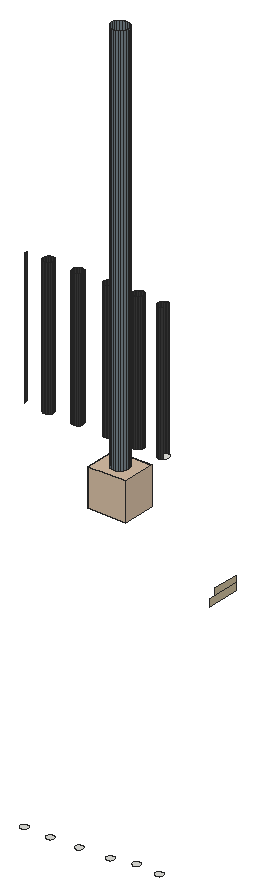
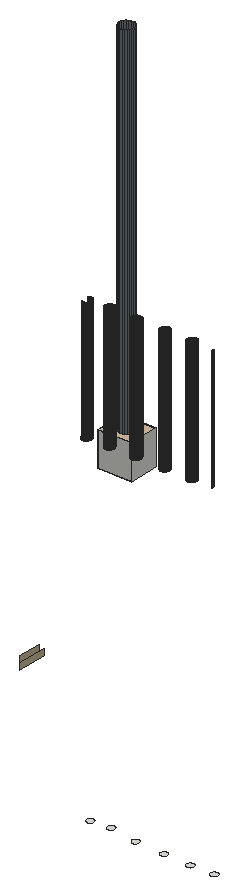
# SketchUp Ruby script. Lengths in inches.
U = 1.inch
M = Sketchup.active_model
def pt(a) = Geom::Point3d.new(a.map { |v| v * U })
def face(e, loops, mat)
  f = e.add_face(loops[0].map { |a| pt(a) })
  loops[1..].each { |l| e.add_face(l.map { |a| pt(a) }).erase! }
  f.material = f.back_material = mat if mat
  f
end
# faces: each face lists its corners as indices into pts; further lists are holes
def faces(e, pts, list, mat = nil) = list.each { |f| face(e, (f[0].is_a?(Array) ? f : [f]).map { |l| l.map { |i| pts[i] } }, mat) }
# xy, xz, yz: faces in a plane at the given z, y or x. An outline is a flat list of corners, or four numbers for a rectangle; further outlines are holes
def ring(l) = l.size == 4 ? [[l[0], l[1]], [l[2], l[1]], [l[2], l[3]], [l[0], l[3]]] : l.each_slice(2).to_a
def flat(e, list, mat, &to3) = list.each { |f| face(e, (f[0].is_a?(Array) ? f : [f]).map { |l| ring(l).map { |u, v| to3.(u, v) } }, mat) }
def xy(e, z, list, mat = nil) = flat(e, list, mat) { |x, y| [x, y, z] }
def xz(e, y, list, mat = nil) = flat(e, list, mat) { |x, z| [x, y, z] }
def yz(e, x, list, mat = nil) = flat(e, list, mat) { |y, z| [x, y, z] }
def lines(e, pts, list) = list.each { |a, b| e.add_line(pt(pts[a]), pt(pts[b])) }
# prism: a flat outline (further loops are holes) pulled along v
def prism(e, loops, v, mat = nil)
  f = face(e, loops, mat); d = Geom::Vector3d.new(v.map { |x| x * U })
  f.pushpull(f.normal.samedirection?(d) ? d.length : -d.length)
end
def box(e, o, s, mat = nil) = prism(e, [[o, [o[0] + s[0], o[1], o[2]], [o[0] + s[0], o[1] + s[1], o[2]], [o[0], o[1] + s[1], o[2]]]], [0, 0, s[2]], mat)
def at(x, y, z, deg = 0) = Geom::Transformation.translation(pt([x, y, z])) * Geom::Transformation.rotation(ORIGIN, Z_AXIS, deg.degrees)
def axes(o, x, y, z) = Geom::Transformation.new([*x, 0, *y, 0, *z, 0, *pt(o).to_a, 1])
def part(name) = M.definitions.add(name)
# library, detail: a bought-in or finely detailed component or shape, given as its bounding box
def library(name, o, s) = part(name).tap { |d| box(d.entities, o, s) }
def detail(e, o, s) = box(e.add_group.entities, o, s)
def put(e, d, t, mat = nil) = e.add_instance(d, t).tap { |i| i.material = mat if mat }
def group(e, t, mat = nil) = e.add_group.tap { |g| g.transformation = t; g.material = mat if mat }.entities
root = M.entities
M.materials.add("[Color M07]").color = [58, 58, 58]
M.materials.add("[Formica Laminate Light]").color = [213, 189, 164]
M.materials.add("[Formica Speckled Grey]").color = [112, 125, 132]
M.materials.add("[Quartz Light Brown]").color = [199, 184, 152]
xy(root,298.96,[[100.78,91.87,100.96,91.89,101.125,91.96,101.27,92.07,101.375,92.21,101.44,92.38,101.47,92.56,101.44,92.73,101.375,92.9,101.27,93.04,101.125,93.15,100.96,93.22,100.78,93.24,100.6,93.22,100.4375,93.15,100.29,93.04,100.18,92.9,100.12,92.73,100.09,92.56,100.12,92.38,100.18,92.21,100.29,92.07,100.4375,91.96,100.6,91.89]])
xy(root,299.02,[[95.78,91.87,95.96,91.89,96.125,91.96,96.27,92.07,96.375,92.21,96.44,92.38,96.47,92.56,96.44,92.73,96.375,92.9,96.27,93.04,96.125,93.15,95.96,93.22,95.78,93.24,95.6,93.22,95.4375,93.15,95.29,93.04,95.18,92.9,95.12,92.73,95.09,92.56,95.12,92.38,95.18,92.21,95.29,92.07,95.4375,91.96,95.6,91.89]])
xy(root,299.14,[[106.34,91.87,106.52,91.89,106.6875,91.96,106.83,92.07,106.9375,92.21,107.01,92.38,107.03,92.56,107.01,92.73,106.9375,92.9,106.83,93.04,106.6875,93.15,106.52,93.22,106.34,93.24,106.16,93.22,106,93.15,105.86,93.04,105.75,92.9,105.68,92.73,105.65,92.56,105.68,92.38,105.75,92.21,105.86,92.07,106,91.96,106.16,91.89]])
xy(root,299.39,[[112.34,91.87,112.52,91.89,112.6875,91.96,112.83,92.07,112.9375,92.21,113.01,92.38,113.03,92.56,113.01,92.73,112.9375,92.9,112.83,93.04,112.6875,93.15,112.52,93.22,112.34,93.24,112.16,93.22,112,93.15,111.86,93.04,111.75,92.9,111.68,92.73,111.65,92.56,111.68,92.38,111.75,92.21,111.86,92.07,112,91.96,112.16,91.89]])
xy(root,299.96,[[121.84,91.87,122.02,91.89,122.1875,91.96,122.33,92.07,122.4375,92.21,122.51,92.38,122.53,92.56,122.51,92.73,122.4375,92.9,122.33,93.04,122.1875,93.15,122.02,93.22,121.84,93.24,121.66,93.22,121.5,93.15,121.36,93.04,121.25,92.9,121.18,92.73,121.15,92.56,121.18,92.38,121.25,92.21,121.36,92.07,121.5,91.96,121.66,91.89]])
xy(root,300.16,[[117.47,91.87,117.64,91.89,117.8125,91.96,117.95,92.07,118.0625,92.21,118.13,92.38,118.15,92.56,118.13,92.73,118.0625,92.9,117.95,93.04,117.8125,93.15,117.64,93.22,117.47,93.24,117.29,93.22,117.125,93.15,116.98,93.04,116.87,92.9,116.8,92.73,116.78,92.56,116.8,92.38,116.87,92.21,116.98,92.07,117.125,91.96,117.29,91.89]])
xy(root,365.02,[[115.36,83.42,122.61,89.73]],"[Formica Laminate Light]")
xy(root,372.27,[[119,85,118.58,85.06,118.1875,85.22,117.85,85.48,117.59,85.82,117.43,86.21,117.375,86.63,117.43,87.05,117.59,87.44,117.85,87.78,118.1875,88.04,118.58,88.2,119,88.25,119.42,88.2,119.8125,88.04,120.15,87.78,120.41,87.44,120.57,87.05,120.625,86.63,120.57,86.21,120.41,85.82,120.15,85.48,119.8125,85.22,119.42,85.06],[100.02,92.0625,99.77,92.1,99.52,92.2,99.32,92.35,99.16,92.5625,99.06,92.8,99.02,93.0625,99.06,93.32,99.16,93.5625,99.32,93.77,99.52,93.93,99.77,94.03,100.02,94.0625,100.28,94.03,100.52,93.93,100.73,93.77,100.89,93.5625,100.99,93.32,101.02,93.0625,100.99,92.8,100.89,92.5625,100.73,92.35,100.52,92.2,100.28,92.1],[105.71,92.0625,105.45,92.1,105.21,92.2,105,92.35,104.85,92.5625,104.75,92.8,104.71,93.0625,104.75,93.32,104.85,93.5625,105,93.77,105.21,93.93,105.45,94.03,105.71,94.0625,105.97,94.03,106.21,93.93,106.42,93.77,106.58,93.5625,106.68,93.32,106.71,93.0625,106.68,92.8,106.58,92.5625,106.42,92.35,106.21,92.2,105.97,92.1],[111.77,92.0625,111.52,92.1,111.27,92.2,111.07,92.35,110.91,92.5625,110.81,92.8,110.77,93.0625,110.81,93.32,110.91,93.5625,111.07,93.77,111.27,93.93,111.52,94.03,111.77,94.0625,112.03,94.03,112.27,93.93,112.48,93.77,112.64,93.5625,112.74,93.32,112.77,93.0625,112.74,92.8,112.64,92.5625,112.48,92.35,112.27,92.2,112.03,92.1],[117.4,92.0625,117.14,92.1,116.9,92.2,116.69,92.35,116.53,92.5625,116.43,92.8,116.4,93.0625,116.43,93.32,116.53,93.5625,116.69,93.77,116.9,93.93,117.14,94.03,117.4,94.0625,117.66,94.03,117.9,93.93,118.11,93.77,118.27,93.5625,118.37,93.32,118.4,93.0625,118.37,92.8,118.27,92.5625,118.11,92.35,117.9,92.2,117.66,92.1],
  [122.21,92.0625,121.95,92.1,121.71,92.2,121.5,92.35,121.35,92.5625,121.25,92.8,121.21,93.0625,121.25,93.32,121.35,93.5625,121.5,93.77,121.71,93.93,121.95,94.03,122.21,94.0625,122.47,94.03,122.71,93.93,122.92,93.77,123.08,93.5625,123.18,93.32,123.21,93.0625,123.18,92.8,123.08,92.5625,122.92,92.35,122.71,92.2,122.47,92.1]])
xy(root,372.27,[[[115.36,83.42,122.61,89.73],[119,85,118.58,85.06,118.1875,85.22,117.85,85.48,117.59,85.82,117.43,86.21,117.375,86.63,117.43,87.05,117.59,87.44,117.85,87.78,118.1875,88.04,118.58,88.2,119,88.25,119.42,88.2,119.8125,88.04,120.15,87.78,120.41,87.44,120.57,87.05,120.625,86.63,120.57,86.21,120.41,85.82,120.15,85.48,119.8125,85.22,119.42,85.06]]],"[Formica Laminate Light]")
xz(root,83.42,[[115.36,365.02,122.61,372.27]],"[Formica Laminate Light]")
xz(root,89.73,[[115.36,365.02,122.61,372.27]])
yz(root,115.36,[[83.42,365.02,89.73,372.27]])
yz(root,119.37,[[107.85,338.67,114.1,339.99],[109.1,339.99,114.1,341.31]],"[Quartz Light Brown]")
yz(root,122.61,[[83.42,365.02,89.73,372.27]],"[Formica Laminate Light]")
p = [[118.58,85.06,372.27],[119,85,372.27],[119,85,448.43],[118.58,85.06,448.43],[119.42,85.06,372.27],[119.42,85.06,448.43],
  [118.1875,85.22,372.27],[118.1875,85.22,448.43],[119.8125,85.22,372.27],[119.8125,85.22,448.43],[117.85,85.48,372.27],[117.85,85.48,448.43],
  [120.15,85.48,372.27],[120.15,85.48,448.43],[117.59,85.82,372.27],[117.59,85.82,448.43],[120.41,85.82,372.27],[120.41,85.82,448.43],
  [117.43,86.21,372.27],[117.43,86.21,448.43],[120.57,86.21,372.27],[120.57,86.21,448.43],[117.375,86.63,372.27],[117.375,86.63,448.43],
  [120.625,86.63,372.27],[120.625,86.63,448.43],[117.43,87.05,372.27],[117.43,87.05,448.43],[120.57,87.05,372.27],[120.57,87.05,448.43],
  [117.59,87.44,372.27],[117.59,87.44,448.43],[120.41,87.44,372.27],[120.41,87.44,448.43],[117.85,87.78,372.27],[117.85,87.78,448.43],
  [120.15,87.78,372.27],[120.15,87.78,448.43],[118.1875,88.04,372.27],[118.1875,88.04,448.43],[119.8125,88.04,372.27],[119.8125,88.04,448.43],
  [118.58,88.2,372.27],[118.58,88.2,448.43],[119.42,88.2,372.27],[119.42,88.2,448.43],[119,88.25,372.27],[119,88.25,448.43],
  [99.52,92.2,372.27],[99.77,92.1,372.27],[99.77,92.1,398.46],[99.52,92.2,398.46],[100.02,92.0625,372.27],[100.02,92.0625,398.46],
  [100.28,92.1,372.27],[100.28,92.1,398.46],[100.52,92.2,372.27],[100.52,92.2,398.46],[105.21,92.2,372.27],[105.45,92.1,372.27],
  [105.45,92.1,398.52],[105.21,92.2,398.52],[105.71,92.0625,372.27],[105.71,92.0625,398.52],[105.97,92.1,372.27],[105.97,92.1,398.52],
  [106.21,92.2,372.27],[106.21,92.2,398.52],[111.27,92.2,372.27],[111.52,92.1,372.27],[111.52,92.1,398.52],[111.27,92.2,398.52],
  [111.77,92.0625,372.27],[111.77,92.0625,398.52],[112.03,92.1,372.27],[112.03,92.1,398.52],[112.27,92.2,372.27],[112.27,92.2,398.52],
  [116.9,92.2,372.27],[117.14,92.1,372.27],[117.14,92.1,398.65],[116.9,92.2,398.65],[117.4,92.0625,372.27],[117.4,92.0625,398.65],
  [117.66,92.1,372.27],[117.66,92.1,398.65],[117.9,92.2,372.27],[117.9,92.2,398.65],[121.71,92.2,372.27],[121.95,92.1,372.27],
  [121.95,92.1,398.4],[121.71,92.2,398.4],[122.21,92.0625,372.27],[122.21,92.0625,398.4],[122.47,92.1,372.27],[122.47,92.1,398.4],
  [122.71,92.2,372.27],[122.71,92.2,398.4],[99.32,92.35,372.27],[99.32,92.35,398.46],[100.73,92.35,372.27],[100.73,92.35,398.46],
  [105,92.35,372.27],[105.1,92.28,398.52],[105,92.35,398.52],[106.42,92.35,372.27],[106.42,92.35,398.52],[106.32,92.28,398.52],
  [111.07,92.35,372.27],[111.17,92.28,398.52],[111.07,92.35,398.52],[112.48,92.35,372.27],[112.48,92.35,398.52],[112.38,92.28,398.52],
  [116.69,92.35,372.27],[116.69,92.35,398.65],[118.11,92.35,372.27],[118.11,92.35,398.65],[121.5,92.35,372.27],[121.5,92.35,398.4],
  [99.16,92.5625,372.27],[99.16,92.5625,398.46],[100.89,92.5625,372.27],[100.89,92.5625,398.46],[104.85,92.5625,372.27],[104.85,92.5625,398.52],
  [106.58,92.5625,372.27],[106.58,92.5625,398.52],[110.91,92.5625,372.27],[110.91,92.5625,398.52],[112.64,92.5625,372.27],[112.64,92.5625,398.52],
  [116.53,92.5625,372.27],[116.53,92.5625,398.65],[118.27,92.5625,372.27],[118.27,92.5625,398.65],[121.35,92.5625,372.27],[121.35,92.5625,398.4],
  [99.06,92.8,372.27],[99.06,92.8,398.46],[100.99,92.8,372.27],[100.99,92.8,398.46],[104.75,92.8,372.27],[104.75,92.8,398.52],
  [106.68,92.8,372.27],[106.68,92.8,398.52],[110.81,92.8,372.27],[110.81,92.8,398.52],[112.74,92.8,372.27],[112.74,92.8,398.52],
  [116.43,92.8,372.27],[116.43,92.8,398.65],[118.37,92.8,372.27],[118.37,92.8,398.65],[121.25,92.8,372.27],[121.25,92.8,398.4],
  [95.62,92.8,372.27],[95.65,93.0625,372.27],[95.65,93.0625,398.15],[95.62,92.8,398.15],[99.02,93.0625,372.27],[99.02,93.0625,398.46],
  [101.02,93.0625,372.27],[101.02,93.0625,398.46],[104.71,93.0625,372.27],[104.71,93.0625,398.52],[106.71,93.0625,372.27],[106.71,93.0625,398.52],
  [110.77,93.0625,372.27],[110.77,93.0625,398.52],[112.77,93.0625,372.27],[112.77,93.0625,398.52],[116.4,93.0625,372.27],[116.4,93.0625,398.65],
  [118.4,93.0625,372.27],[118.4,93.0625,398.65],[121.21,93.0625,372.27],[121.21,93.0625,398.4],[95.62,93.32,372.27],[95.62,93.32,398.15],
  [99.06,93.32,372.27],[99.06,93.32,398.46],[100.99,93.32,372.27],[100.99,93.32,398.46],[104.75,93.32,372.27],[104.75,93.32,398.52],
  [106.68,93.32,372.27],[106.68,93.32,398.52],[110.81,93.32,372.27],[110.81,93.32,398.52],[112.74,93.32,372.27],[112.74,93.32,398.52],
  [116.43,93.32,372.27],[116.43,93.32,398.65],[118.37,93.32,372.27],[118.37,93.32,398.65],[121.25,93.32,372.27],[121.25,93.32,398.4],
  [99.16,93.5625,372.27],[99.16,93.5625,398.46],[100.89,93.5625,372.27],[100.89,93.5625,398.46],[104.85,93.5625,372.27],[104.85,93.5625,398.52],
  [106.58,93.5625,372.27],[106.58,93.5625,398.52],[110.91,93.5625,372.27],[110.91,93.5625,398.52],[112.64,93.5625,372.27],[112.64,93.5625,398.52],
  [116.53,93.5625,372.27],[116.53,93.5625,398.65],[118.27,93.5625,372.27],[118.27,93.5625,398.65],[121.35,93.5625,372.27],[121.35,93.5625,398.4],
  [99.32,93.77,372.27],[99.32,93.77,398.46],[100.73,93.77,372.27],[100.73,93.77,398.46],[105,93.77,372.27],[105,93.77,398.52],
  [106.42,93.77,372.27],[106.42,93.77,398.52],[111.07,93.77,372.27],[111.07,93.77,398.52],[112.48,93.77,372.27],[112.48,93.77,398.52],
  [116.69,93.77,372.27],[116.69,93.77,398.65],[118.11,93.77,372.27],[118.11,93.77,398.65],[121.5,93.77,372.27],[121.5,93.77,398.4],
  [99.52,93.93,372.27],[99.52,93.93,398.46],[99.52,93.93,388.09],[99.52,93.93,385.79],[100.52,93.93,372.27],[100.52,93.93,385.79],
  [100.52,93.93,388.09],[100.52,93.93,398.46],[105.21,93.93,372.27],[105.21,93.93,398.52],[105.21,93.93,388.09],[105.21,93.93,385.79],
  [106.21,93.93,372.27],[106.21,93.93,385.79],[106.21,93.93,388.09],[106.21,93.93,398.52],[111.27,93.93,372.27],[111.27,93.93,398.52],
  [111.27,93.93,388.09],[111.27,93.93,385.79],[112.27,93.93,372.27],[112.27,93.93,385.79],[112.27,93.93,388.09],[112.27,93.93,398.52],
  [116.9,93.93,372.27],[116.9,93.93,398.65],[116.9,93.93,388.09],[116.9,93.93,385.79],[117.9,93.93,372.27],[117.9,93.93,385.79],
  [117.9,93.93,388.09],[117.9,93.93,398.65],[121.71,93.93,372.27],[121.71,93.93,398.4],[121.71,93.93,388.09],[121.71,93.93,385.79],
  [99.77,94.03,372.27],[99.77,94.03,398.46],[100.28,94.03,372.27],[100.28,94.03,398.46],[105.45,94.03,372.27],[105.45,94.03,398.52],
  [105.97,94.03,372.27],[105.97,94.03,398.52],[111.52,94.03,372.27],[111.52,94.03,398.52],[112.03,94.03,372.27],[112.03,94.03,398.52],
  [117.14,94.03,372.27],[117.14,94.03,398.65],[117.66,94.03,372.27],[117.66,94.03,398.65],[121.95,94.03,372.27],[121.95,94.03,398.4],
  [100.02,94.0625,372.27],[100.02,94.0625,398.46],[105.71,94.0625,372.27],[105.71,94.0625,398.52],[111.77,94.0625,372.27],[111.77,94.0625,398.52],
  [117.4,94.0625,372.27],[117.4,94.0625,398.65],[122.21,94.0625,372.27],[122.21,94.0625,398.4],[122.47,94.03,372.27],[122.47,94.03,398.4]]
faces(root,p,[[0,1,2,3],[1,4,5,2],[6,0,3,7],[4,8,9,5],[10,6,7,11],[8,12,13,9],[14,10,11,15],[12,16,17,13],
  [18,14,15,19],[16,20,21,17],[22,18,19,23],[20,24,25,21],[26,22,23,27],[24,28,29,25],[30,26,27,31],[28,32,33,29],
  [34,30,31,35],[32,36,37,33],[38,34,35,39],[36,40,41,37],[42,38,39,43],[40,44,45,41],[46,42,43,47],[44,46,47,45]],"[Formica Speckled Grey]")
faces(root,p,[[48,49,50,51],[49,52,53,50],[52,54,55,53],[54,56,57,55],[58,59,60,61],[59,62,63,60],[62,64,65,63],[64,66,67,65],
  [68,69,70,71],[69,72,73,70],[72,74,75,73],[74,76,77,75],[78,79,80,81],[79,82,83,80],[82,84,85,83],[84,86,87,85],
  [88,89,90,91],[89,92,93,90],[92,94,95,93],[94,96,97,95],[98,48,51,99],[56,100,101,57],[102,58,61,103,104],[66,105,106,107,67],
  [108,68,71,109,110],[76,111,112,113,77],[114,78,81,115],[86,116,117,87],[118,88,91,119],[120,98,99,121],[100,122,123,101],[124,102,104,125],
  [105,126,127,106],[128,108,110,129],[111,130,131,112],[132,114,115,133],[116,134,135,117],[136,118,119,137],[138,120,121,139],[122,140,141,123],
  [142,124,125,143],[126,144,145,127],[146,128,129,147],[130,148,149,131],[150,132,133,151],[134,152,153,135],[154,136,137,155],[156,157,158,159],
  [160,138,139,161],[140,162,163,141],[164,142,143,165],[144,166,167,145],[168,146,147,169],[148,170,171,149],[172,150,151,173],[152,174,175,153],
  [176,154,155,177],[157,178,179,158],[180,160,161,181],[162,182,183,163],[184,164,165,185],[166,186,187,167],[188,168,169,189],[170,190,191,171],
  [192,172,173,193],[174,194,195,175],[196,176,177,197],[198,180,181,199],[182,200,201,183],[202,184,185,203],[186,204,205,187],[206,188,189,207],
  [190,208,209,191],[210,192,193,211],[194,212,213,195],[214,196,197,215],[216,198,199,217],[200,218,219,201],[220,202,203,221],[204,222,223,205],
  [224,206,207,225],[208,226,227,209],[228,210,211,229],[212,230,231,213],[232,214,215,233],[234,216,217,235,236,237],[218,238,239,240,241,219],[242,220,221,243,244,245],
  [222,246,247,248,249,223],[250,224,225,251,252,253],[226,254,255,256,257,227],[258,228,229,259,260,261],[230,262,263,264,265,231],[266,232,233,267,268,269],[270,234,237,236,235,271],[238,272,273,241,240,239],
  [274,242,245,244,243,275],[246,276,277,249,248,247],[278,250,253,252,251,279],[254,280,281,257,256,255],[282,258,261,260,259,283],[262,284,285,265,264,263],[286,266,269,268,267,287],[288,270,271,289],
  [272,288,289,273],[290,274,275,291],[276,290,291,277],[292,278,279,293],[280,292,293,281],[294,282,283,295],[284,294,295,285],[296,286,287,297],
  [298,296,297,299]],"[Color M07]")
